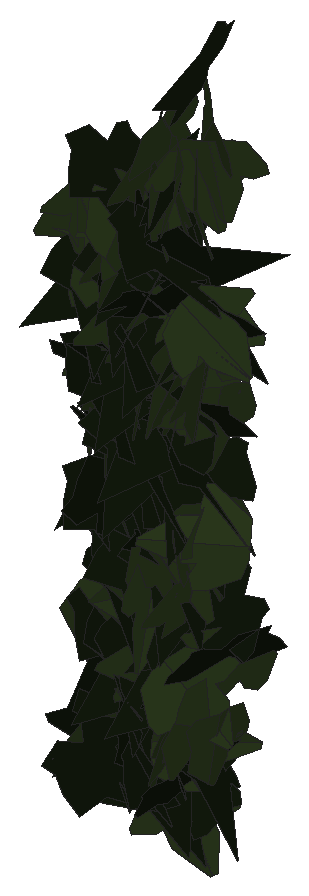
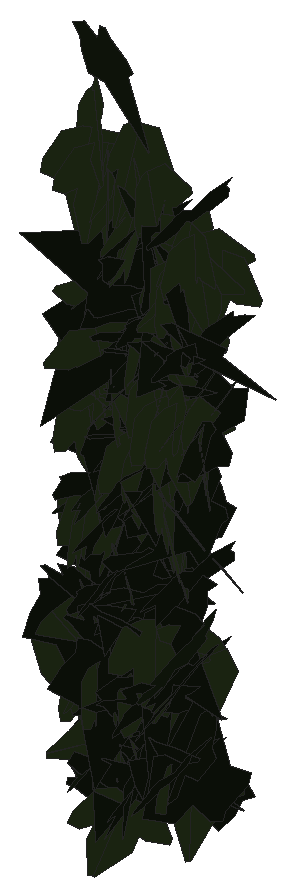
# SketchUp Ruby script. Lengths in inches.
U = 1.inch
M = Sketchup.active_model
def pt(a) = Geom::Point3d.new(a.map { |v| v * U })
def face(e, loops, mat)
  f = e.add_face(loops[0].map { |a| pt(a) })
  loops[1..].each { |l| e.add_face(l.map { |a| pt(a) }).erase! }
  f.material = f.back_material = mat if mat
  f
end
# faces: each face lists its corners as indices into pts; further lists are holes
def faces(e, pts, list, mat = nil) = list.each { |f| face(e, (f[0].is_a?(Array) ? f : [f]).map { |l| l.map { |i| pts[i] } }, mat) }
# xy, xz, yz: faces in a plane at the given z, y or x. An outline is a flat list of corners, or four numbers for a rectangle; further outlines are holes
def ring(l) = l.size == 4 ? [[l[0], l[1]], [l[2], l[1]], [l[2], l[3]], [l[0], l[3]]] : l.each_slice(2).to_a
def flat(e, list, mat, &to3) = list.each { |f| face(e, (f[0].is_a?(Array) ? f : [f]).map { |l| ring(l).map { |u, v| to3.(u, v) } }, mat) }
def xy(e, z, list, mat = nil) = flat(e, list, mat) { |x, y| [x, y, z] }
def xz(e, y, list, mat = nil) = flat(e, list, mat) { |x, z| [x, y, z] }
def yz(e, x, list, mat = nil) = flat(e, list, mat) { |y, z| [x, y, z] }
def lines(e, pts, list) = list.each { |a, b| e.add_line(pt(pts[a]), pt(pts[b])) }
# prism: a flat outline (further loops are holes) pulled along v
def prism(e, loops, v, mat = nil)
  f = face(e, loops, mat); d = Geom::Vector3d.new(v.map { |x| x * U })
  f.pushpull(f.normal.samedirection?(d) ? d.length : -d.length)
end
def box(e, o, s, mat = nil) = prism(e, [[o, [o[0] + s[0], o[1], o[2]], [o[0] + s[0], o[1] + s[1], o[2]], [o[0], o[1] + s[1], o[2]]]], [0, 0, s[2]], mat)
def at(x, y, z, deg = 0) = Geom::Transformation.translation(pt([x, y, z])) * Geom::Transformation.rotation(ORIGIN, Z_AXIS, deg.degrees)
def axes(o, x, y, z) = Geom::Transformation.new([*x, 0, *y, 0, *z, 0, *pt(o).to_a, 1])
def part(name) = M.definitions.add(name)
# library, detail: a bought-in or finely detailed component or shape, given as its bounding box
def library(name, o, s) = part(name).tap { |d| box(d.entities, o, s) }
def detail(e, o, s) = box(e.add_group.entities, o, s)
def put(e, d, t, mat = nil) = e.add_instance(d, t).tap { |i| i.material = mat if mat }
def group(e, t, mat = nil) = e.add_group.tap { |g| g.transformation = t; g.material = mat if mat }.entities
root = M.entities
M.materials.add("efeu1").color = [18, 25, 13]
M.materials.add("efeu2").color = [43, 57, 29]
c1 = part("ivyleaf_10")
p = [[0,0.5,-0.03],[-0.0625,2.02,-0.43],[-0.19,2.01,-0.46],[-0.54,1.05,-0.29],[-0.52,0.625,-0.18],[-0.83,0.76,-0.28],
  [-1.16,0.64,-0.33],[-1.15,0.33,-0.24],[-0.77,-0.39,0.02],[-0.3,-0.51,0.16],[0.04,-0.48,0.23],[-0.02,2.01,-0.4375],
  [-0.06,2.01,-0.43],[0.04,-0.49,0.23],[0.67,-0.49,0.14],[1.38,0.36,-0.2],[1.375,0.51,-0.24],[0.81,0.65,-0.19],
  [0.62,0.59,-0.15],[0.6,1.09,-0.28],[0.5,1.23,-0.31]]
faces(c1.entities,p,[[0,1,2,3,4,5,6,7,8,9,10],[11,12,0,13,14,15,16,17,18,19,20]],"efeu2")
c2 = part("ivyleaf_9")
p = [[1.54,2.16,1.25],[1.36,2.04,1.19],[-0.21,0.99,0.68],[-0.71,1.11,0.82],[-0.85,0.86,0.67],[-0.8,0.17,0.21],
  [-0.9,-0.01,0.1],[-0.67,-0.16,-0.02],[-0.08,-0.08,-0.05],[-0.03,-0.6,-0.4],[0.65,-0.88,-0.66],[0.83,-0.6,-0.49],
  [1.29,-0.42,-0.43],[1.8125,-0.07,-0.26],[1.21,0.44,0.15]]
faces(c2.entities,p,[[0,1,2,3,4,5,6,7,8,9,10,11,12,13,14]],"efeu1")
put(root,c1,axes([29.85,223.89,228.47],[0.26716,-0.40382,0.12471],[0.14043,-0.05434,-0.47679],[0.39863,0.28978,0.08438]))
put(root,c2,axes([29.9,224.07,223.78],[0.38812,0.14363,0.28059],[-0.26637,-0.08852,0.41377],[0.16854,-0.47067,0.00781]))
put(root,c2,axes([30.25,223.96,230],[-0.48861,-0.00888,0.10574],[-0.10448,-0.04687,-0.48671],[0.01855,-0.49772,0.04395]))
put(root,c1,axes([30.0625,223.85,223.93],[-0.17024,-0.46382,-0.07671],[0.02705,0.07179,-0.49408],[0.46935,-0.17238,0.00065]))
put(root,c2,axes([29.85,224.13,226.97],[0.10622,-0.46612,-0.14646],[0.00388,0.15068,-0.47674],[0.48857,0.10014,0.03563]))
put(root,c1,axes([30.12,223.68,231.06],[-0.21352,-0.44848,0.05721],[0.00729,-0.06668,-0.49548],[0.45206,-0.21076,0.03501]))
put(root,c1,axes([30.04,223.53,230.84],[-0.40589,-0.26421,-0.12429],[0.13274,0.0226,-0.48153],[0.26006,-0.42389,0.0518]))
put(root,c2,axes([29.95,223.95,230.02],[-0.04725,-0.49721,0.02346],[-0.00355,-0.02323,-0.49945],[0.49775,-0.04737,-0.00133]))
put(root,c1,axes([30.15,224,228.85],[-0.17671,-0.4661,0.03897],[0.00687,-0.04424,-0.49799],[0.46768,-0.17547,0.02204]))
put(root,c2,axes([30.29,224,227.68],[-0.46968,0.13341,-0.10772],[0.09572,-0.05663,-0.48747],[-0.14226,-0.47854,0.02766]))
put(root,c2,axes([29.84,223.87,227.83],[0.48976,-0.09852,0.0208],[0.01861,-0.01292,-0.49949],[0.09896,0.49003,-0.00899]))
put(root,c1,axes([30.11,224.2,227.48],[0.26689,-0.41548,0.07837],[0.06087,-0.05396,-0.49334],[0.41841,0.27288,0.02178]))
put(root,c2,axes([30.01,224.27,224.2],[0.04138,-0.4968,0.03841],[0.00516,-0.03812,-0.49852],[0.49826,0.04165,0.00197]))
put(root,c2,axes([30,223.95,225.52],[0.19361,-0.40981,-0.21112],[-0.0449,0.21113,-0.45101],[0.4588,0.1936,0.04495]))
put(root,c2,axes([29.99,223.72,228.8125],[0.23455,-0.4415,-0.00777],[-0.00599,0.00562,-0.49993],[0.44153,0.23461,-0.00265]))
put(root,c1,axes([30.28,223.74,230.73],[-0.4002,-0.2934,0.06127],[0.03933,-0.15274,-0.47447],[0.29714,-0.37495,0.14533]))
put(root,c2,axes([30.32,223.53,230.0625],[0.03232,-0.06399,0.49483],[0.07202,0.49128,0.05883],[-0.49373,0.06747,0.04098]))
put(root,c2,axes([29.98,224.3125,225.68],[0.06322,-0.42118,0.26193],[0.12686,-0.24154,-0.419],[0.47949,0.11944,0.07632]))
put(root,c1,axes([29.96,223.73,225.59],[-0.25331,-0.06923,-0.42549],[0.41686,0.08639,-0.26223],[0.10982,-0.48759,0.01396]))
put(root,c2,axes([29.87,223.64,228.7],[0.34275,-0.11962,0.34382],[0.35985,0.03996,-0.34483],[0.05502,0.48383,0.11349]))
put(root,c2,axes([30,224.1,224.17],[-0.02108,-0.21411,0.45135],[0.26555,-0.38744,-0.17139],[0.42313,0.23248,0.13005]))
put(root,c1,axes([30.5,223.4,227.48],[-0.26448,0.22755,0.35815],[-0.26964,0.23574,-0.34889],[-0.32764,-0.37769,-0.00198]))
put(root,c1,axes([30.35,223.67,231.18],[-0.48752,0.09896,-0.0503],[0.0301,-0.10022,-0.48893],[-0.10685,-0.47975,0.09176]))
put(root,c2,axes([30.61,224.11,224.21],[-0.48401,-0.0498,0.11513],[-0.11153,-0.03915,-0.48583],[0.0574,-0.49597,0.02679]))
put(root,c1,axes([30.39,224.01,227.875],[0.14948,-0.47446,-0.05045],[-0.00197,0.05225,-0.49726],[0.47713,0.14886,0.01375]))
put(root,c1,axes([30.42,224.04,228.82],[-0.1036,-0.489,0.01221],[0.00279,-0.01307,-0.49982],[0.48914,-0.1035,0.00543]))
put(root,c1,axes([30.42,223.73,230.45],[0.00872,-0.49912,-0.02842],[-0.01446,0.02816,-0.499],[0.49971,0.00952,-0.01394]))
put(root,c2,axes([30.2,223.74,228.73],[0.48839,-0.00888,-0.10674],[-0.10541,0.04843,-0.48636],[0.01898,0.49757,0.04543]))
put(root,c2,axes([30.16,224.1,225.17],[0.11367,-0.47837,0.09079],[0.01033,-0.09084,-0.49157],[0.4868,0.11363,-0.01077]))
put(root,c2,axes([30.15,223.86,228.99],[0.262,-0.42456,-0.0333],[-0.01741,0.02839,-0.49889],[0.4255,0.26258,0.00009]))
put(root,c2,axes([30.26,223.49,227.01],[0.00549,-0.10348,0.48914],[0.35762,0.34267,0.06848],[-0.3494,0.3491,0.07778]))
put(root,c1,axes([30.48,224.07,225.78],[-0.3492,-0.35782,-0.00487],[0.00269,0.00417,-0.49998],[0.35785,-0.3492,-0.00099]))
put(root,c2,axes([30.67,224,225.91],[0.09889,0.1002,-0.47977],[-0.31893,-0.35849,-0.1406],[-0.37216,0.33383,-0.00699]))
put(root,c2,axes([30.23,223.68,231.64],[0.14225,-0.45982,-0.13539],[-0.01017,0.1383,-0.48038],[0.47923,0.13943,0.03]))
put(root,c2,axes([30.125,223.42,223.88],[0.04061,-0.07147,-0.4932],[0.2929,0.40377,-0.03439],[0.40319,-0.28612,0.07466]))
put(root,c1,axes([30.52,224.01,229.18],[-0.09335,-0.49031,0.02963],[0.00691,-0.03147,-0.49896],[0.49116,-0.09275,0.01266]))
put(root,c2,axes([30.51,223.81,223.91],[0.02181,-0.22135,0.44781],[0.15316,0.42961,0.20489],[-0.47547,0.12823,0.08654]))
put(root,c1,axes([30.56,223.63,229.61],[-0.13993,-0.47976,0.01569],[0.0233,-0.02311,-0.49892],[0.47945,-0.1389,0.02882]))
put(root,c2,axes([30.68,224.27,224.99],[-0.40527,-0.24121,0.16604],[-0.09604,-0.15833,-0.46444],[0.27664,-0.40835,0.082]))
put(root,c2,axes([30.37,223.98,228.04],[0.05257,-0.49722,-0.0025],[-0.00865,0.0016,-0.49992],[0.49715,0.0526,-0.00843]))
put(root,c1,axes([30.39,223.91,229.15],[-0.35915,0.21003,-0.27731],[0.21924,-0.1728,-0.41482],[-0.27009,-0.41956,0.03203]))
put(root,c1,axes([30.39,223.48,230.14],[0.47013,0.07326,0.15367],[0.12461,0.15944,-0.45722],[-0.11599,0.4682,0.13165]))
put(root,c2,axes([30.44,224.19,225.07],[-0.03476,-0.49071,0.08941],[-0.01691,-0.08842,-0.49183],[0.4985,-0.03721,-0.01044]))
put(root,c1,axes([30.5625,223.32,230.27],[-0.00824,-0.05377,-0.49703],[0.08859,0.48908,-0.05437],[0.49202,-0.08896,0.00147]))
put(root,c1,axes([30.58,223.28,230.76],[0.05642,0.29166,-0.40218],[0.06515,0.39693,0.29699],[0.49252,-0.08592,0.00679]))
put(root,c2,axes([30.36,224.03,226.74],[-0.06153,-0.23427,-0.43741],[0.22853,0.37785,-0.23452],[0.44044,-0.22879,0.06058]))
put(root,c1,axes([30.71,223.92,225.01],[-0.16641,-0.42959,0.19431],[-0.02515,-0.19767,-0.45858],[0.47082,-0.1624,0.04418]))
put(root,c1,axes([30.64,224.09,228.22],[-0.03781,-0.37581,0.32763],[0.05527,-0.3297,-0.37181],[0.4955,0.0081,0.06647]))
put(root,c2,axes([30.55,223.92,230.21],[-0.14448,-0.47577,0.05257],[-0.00672,-0.05289,-0.49715],[0.47862,-0.14436,0.00889]))
put(root,c2,axes([30.77,223.48,229.63],[0.00242,0.30071,0.39946],[0.00566,0.39942,-0.30072],[-0.49996,0.00598,-0.00147]))
put(root,c2,axes([30.73,223.74,230.63],[0.01415,-0.18521,0.46422],[0.08212,0.45895,0.18061],[-0.49301,0.07113,0.04341]))
put(root,c1,axes([30.8,223.48,228.61],[-0.00758,-0.00903,-0.49986],[-0.12015,0.4853,-0.00695],[0.48529,0.12001,-0.00953]))
put(root,c2,axes([30.43,223.93,227.66],[0.49275,0.08219,0.02097],[-0.02119,-0.00043,0.49955],[0.08213,-0.4932,0.00306]))
put(root,c1,axes([30.74,224.1,228.32],[-0.2251,-0.44479,0.03856],[0.0163,-0.05135,-0.49709],[0.44616,-0.22254,0.03762]))
put(root,c2,axes([30.88,223.9375,229.56],[-0.45407,-0.20365,0.04847],[-0.01998,-0.07309,-0.49423],[0.20838,-0.45076,0.05824]))
put(root,c2,axes([30.77,223.97,229.1],[-0.38053,-0.3241,0.01262],[0.0551,-0.08376,-0.48984],[0.31963,-0.37141,0.09947]))
put(root,c1,axes([30.8,223.76,229.54],[-0.03252,-0.49692,-0.04482],[0.01281,0.04407,-0.49789],[0.49878,-0.03353,0.00986]))
put(root,c2,axes([30.63,224.08,226.37],[-0.21162,-0.4265,-0.15269],[0.14556,0.09557,-0.4687],[0.42899,-0.24282,0.08371]))
put(root,c2,axes([30.8,223.86,228.13],[-0.27431,-0.4157,0.0441],[-0.01646,-0.04197,-0.49796],[0.41771,-0.27464,0.00934]))
put(root,c1,axes([30.875,223.98,228],[-0.27222,-0.41078,0.08458],[-0.01129,-0.09362,-0.49103],[0.41925,-0.26925,0.04169]))
put(root,c1,axes([30.84,223.65,231.67],[0.04783,-0.49698,-0.02694],[0.00162,0.02722,-0.49926],[0.4977,0.04767,0.00421]))
put(root,c2,axes([30.9,223.92,230.8],[-0.41343,-0.28108,0.00832],[-0.00459,-0.00805,-0.49991],[0.28116,-0.41344,0.00407]))
put(root,c2,axes([30.65,224.13,228.11],[0.02881,-0.49897,0.01397],[-0.00038,-0.01402,-0.4998],[0.49917,0.02879,-0.00118]))
put(root,c2,axes([30.99,223.77,224.34],[0.20137,0.02156,-0.45715],[-0.44406,0.13005,-0.18948],[0.11074,0.48231,0.07152]))
put(root,c2,axes([30.6,223.79,228.09],[0.25879,-0.42727,0.02155],[0.00952,-0.01943,-0.49953],[0.42771,0.25896,-0.00192]))
put(root,c2,axes([30.67,223.93,223.78],[0.23012,-0.40585,-0.17982],[-0.07141,0.16606,-0.46618],[0.43812,0.24023,0.01846]))
put(root,c2,axes([30.68,223.83,224.02],[-0.2105,-0.2182,-0.3976],[0.27289,0.28917,-0.30317],[0.36225,-0.34463,-0.00265]))
put(root,c1,axes([30.88,223.72,226.125],[0.07516,0.43946,-0.22634],[-0.02851,-0.22471,-0.44575],[-0.4935,0.07991,-0.00872]))
put(root,c2,axes([31.05,224.3,224.88],[-0.30338,-0.30542,0.25433],[-0.12983,-0.22625,-0.42656],[0.37564,-0.32486,0.05797]))
put(root,c2,axes([31.11,223.4375,230.1],[0.15068,0.44742,-0.16464],[-0.11117,-0.13493,-0.46844],[-0.46361,0.17778,0.05882]))
put(root,c2,axes([31.04,223.92,229.78],[-0.29662,-0.40196,0.02123],[-0.00951,-0.01937,-0.49953],[0.4024,-0.29674,0.00384]))
put(root,c2,axes([30.8,223.7,229.43],[0.29036,-0.36272,-0.18472],[-0.05263,0.19155,-0.45885],[0.40363,0.28591,0.07306]))
put(root,c2,axes([31.11,223.9375,228.36],[-0.39516,-0.28806,0.10426],[-0.0061,-0.16273,-0.47274],[0.30629,-0.37489,0.12509]))
put(root,c1,axes([30.99,223.83,224.31],[0.25783,-0.40652,0.13515],[0.07517,-0.11236,-0.48138],[0.42175,0.26855,0.00318]))
put(root,c1,axes([30.96,223.93,231.27],[-0.32903,0.35299,-0.13092],[0.09468,-0.0907,-0.4825],[-0.36438,-0.34231,-0.00716]))
put(root,c2,axes([31.4,224.19,223.61],[-0.4234,-0.00044,0.26595],[-0.26579,-0.017,-0.42317],[0.00941,-0.49971,0.01416]))
put(root,c2,axes([31.3,223.55,231.68],[-0.37444,0.32957,-0.03431],[0.02075,-0.02835,-0.49876],[-0.3307,-0.37494,0.00755]))
put(root,c1,axes([31.11,223.95,226.6],[0.31279,-0.3849,-0.06334],[-0.03689,0.05164,-0.49596],[0.38833,0.31493,0.0039]))
put(root,c2,axes([31.02,224.24,226.45],[-0.19567,-0.45991,0.01417],[0.01596,-0.02217,-0.49925],[0.45985,-0.19492,0.02336]))
put(root,c1,axes([31.1,223.63,232.24],[-0.05219,-0.42895,-0.25155],[0.05629,0.24621,-0.43152],[0.49407,-0.07336,0.02259]))
put(root,c2,axes([31.13,223.72,226.83],[0.30317,0.3756,-0.13042],[-0.10641,-0.08138,-0.48172],[-0.3831,0.31984,0.03059]))
put(root,c2,axes([31.39,224.18,225.75],[-0.48692,-0.01843,0.11211],[-0.11209,-0.00258,-0.48727],[0.01854,-0.49965,-0.00162]))
put(root,c1,axes([31.13,223.88,228.8],[0.15748,-0.47412,-0.02016],[0.00923,0.02429,-0.49932],[0.47446,0.15689,0.0164]))
put(root,c1,axes([31.03,224.01,223.24],[-0.36431,-0.30487,-0.15597],[0.2026,-0.00828,-0.45704],[0.27609,-0.39621,0.12956]))
put(root,c2,axes([30.93,224.2,226.66],[0.10635,-0.48766,0.02959],[-0.00101,-0.0305,-0.49907],[0.48856,0.10609,-0.00747]))
put(root,c2,axes([31.23,223.78,228.49],[0.30274,0.34621,-0.19619],[-0.18202,-0.09874,-0.4551],[-0.35386,0.34697,0.06625]))
put(root,c1,axes([31.09,223.66,231.32],[-0.06753,0.49241,-0.05453],[0.00521,-0.05433,-0.49701],[-0.49539,-0.06769,0.00221]))
put(root,c2,axes([30.97,224.09,227.41],[0.14219,-0.45593,-0.14802],[-0.01687,0.14954,-0.47681],[0.47906,0.14059,0.02715]))
put(root,c1,axes([31.125,223.86,229.17],[0.13119,-0.36647,0.31383],[0.11585,-0.29178,-0.38915],[0.46837,0.17482,0.00835]))
put(root,c2,axes([30.78,223.84,229.69],[0.34807,-0.27082,0.23559],[0.2465,-0.0582,-0.4311],[0.26093,0.41626,0.093]))
put(root,c2,axes([30.98,223.51,231.11],[0.20732,-0.37921,-0.25143],[-0.02393,0.26683,-0.42217],[0.45436,0.18709,0.09249]))
put(root,c1,axes([30.91,223.63,229.24],[-0.14657,-0.08957,-0.46957],[0.43306,0.18309,-0.1701],[0.20242,-0.45657,0.0239]))
put(root,c1,axes([31.29,223.56,224.49],[0.07626,-0.40591,-0.28181],[-0.02728,0.28126,-0.41249],[0.4934,0.07829,0.02075]))
put(root,c2,axes([31.28,223.8,224.95],[0.17159,0.46818,-0.03697],[-0.00388,-0.03794,-0.49854],[-0.46962,0.17137,-0.00939]))
put(root,c1,axes([31.39,223.41,231.8125],[0.22619,-0.3307,-0.29913],[-0.16815,0.24739,-0.40065],[0.41299,0.28185,0.0007]))
put(root,c1,axes([31.16,223.57,226.63],[-0.43563,-0.12456,-0.21146],[0.20936,0.03619,-0.45261],[0.12806,-0.48288,0.02063]))
put(root,c1,axes([31.29,223.84,229.03],[-0.38224,-0.32218,0.00969],[0.0653,-0.09213,-0.48708],[0.31564,-0.37109,0.11251]))
put(root,c1,axes([31.3,223.72,226.99],[-0.16891,0.45208,0.13075],[-0.06609,0.11476,-0.48214],[-0.46594,-0.18016,0.02099]))
put(root,c1,axes([31.34,224.02,224.85],[0.01782,-0.49957,-0.01062],[-0.00485,0.01046,-0.49987],[0.49966,0.01792,-0.00447]))
put(root,c2,axes([31.375,223.44,223.89],[0.10729,0.47232,0.1241],[0.0286,0.12076,-0.48435],[-0.48751,0.11103,-0.0011]))
put(root,c1,axes([31.36,223.73,226.21],[-0.01523,-0.49973,0.00613],[0.00014,-0.00614,-0.49996],[0.49977,-0.01523,0.00032]))
put(root,c2,axes([31.3,224.18,227.86],[-0.25564,-0.4297,-0.00226],[0.02762,-0.0138,-0.49905],[0.42882,-0.25528,0.03079]))
put(root,c1,axes([31.34,224.07,229.62],[0.33021,0.36995,-0.06402],[-0.08001,-0.01396,-0.49336],[-0.36682,0.33607,0.04998]))
put(root,c1,axes([31.16,223.73,224.125],[0.05199,0.02371,0.49672],[0.19834,0.457,-0.04258],[-0.45602,0.20147,0.03812]))
put(root,c2,axes([31.13,224.0625,227.88],[0.30837,-0.39356,0.0047],[0.04457,0.02899,-0.49716],[0.39105,0.30704,0.05296]))
put(root,c2,axes([31.3,223.88,229.74],[0.46464,0.18166,-0.0333],[-0.03121,-0.01162,-0.49889],[-0.18203,0.46569,0.00054]))
put(root,c1,axes([31.52,223.87,227.18],[-0.26213,-0.42565,0.01034],[-0.00587,-0.00853,-0.49989],[0.42574,-0.2622,-0.00053]))
put(root,c1,axes([31.54,224.02,228.61],[-0.20249,-0.45339,0.05861],[0.00898,-0.06804,-0.49527],[0.45707,-0.19952,0.0357]))
put(root,c1,axes([31.53,223.76,231.87],[-0.34118,-0.35436,-0.08958],[0.09817,0.0292,-0.4894],[0.35208,-0.35153,0.04965]))
put(root,c2,axes([31.81,223.47,233.32],[-0.30752,0.39222,0.0399],[-0.01717,0.03723,-0.49832],[-0.39387,-0.30786,-0.00943]))
put(root,c1,axes([31.8,223.37,231.49],[-0.18213,0.1331,0.44622],[-0.35779,0.26665,-0.22557],[-0.29802,-0.40147,-0.00189]))
put(root,c1,axes([31.83,223.62,232.51],[-0.27082,0.15181,0.39193],[-0.35506,0.16687,-0.30998],[-0.22492,-0.44622,0.01742]))
put(root,c1,axes([31.59,223.65,229.17],[0.13302,-0.47815,-0.06067],[0.01616,0.06732,-0.49518],[0.48171,0.12978,0.03336]))
put(root,c2,axes([31.19,223.58,230.4],[0.19616,-0.07079,0.45443],[0.45949,0.05141,-0.19034],[-0.01978,0.49229,0.08523]))
put(root,c2,axes([31.3125,223.99,224.05],[0.22382,-0.43519,0.10254],[0.05235,-0.08838,-0.48934],[0.44403,0.22978,0.006]))
put(root,c1,axes([31.88,223.77,226.98],[-0.0508,0.13525,0.47867],[-0.32892,-0.37008,0.06966],[0.37313,-0.30782,0.12657]))
put(root,c1,axes([31.55,224.04,227.09],[0.05383,-0.49531,0.04211],[0.13964,-0.02558,-0.47942],[0.47708,0.06338,0.13558]))
put(root,c2,axes([31.84,224.05,226.15],[-0.49949,-0.02028,-0.00972],[0.00986,-0.00328,-0.49989],[0.02021,-0.49958,0.00368]))
put(root,c1,axes([31.7,223.76,232.02],[-0.43722,-0.23983,-0.0364],[0.02913,0.02258,-0.49864],[0.24082,-0.43815,-0.00577]))
put(root,c1,axes([31.46,223.39,225.22],[0.2567,0.29959,0.30716],[0.18972,0.24179,-0.39439],[-0.38485,0.31903,0.01046]))
put(root,c1,axes([31.87,224.06,225.45],[-0.21608,-0.32125,0.3164],[-0.16266,-0.27169,-0.38694],[0.42053,-0.27016,0.0129]))
put(root,c1,axes([31.82,223.65,224.61],[-0.10499,-0.48884,-0.00282],[0.00018,0.00285,-0.49999],[0.48885,-0.10499,-0.00042]))
put(root,c1,axes([31.71,223.24,224.81],[-0.04678,-0.2481,-0.43158],[0.14819,0.40688,-0.24997],[0.47524,-0.1513,0.03546]))
put(root,c1,axes([31.61,223.55,229.92],[0.14963,0.36652,0.30541],[0.12115,0.2804,-0.39585],[-0.46145,0.19246,-0.0049]))
put(root,c2,axes([31.91,223.65,225.64],[0.07334,0.47655,-0.13238],[-0.04117,-0.12749,-0.48172],[-0.49288,0.08156,0.02054]))
